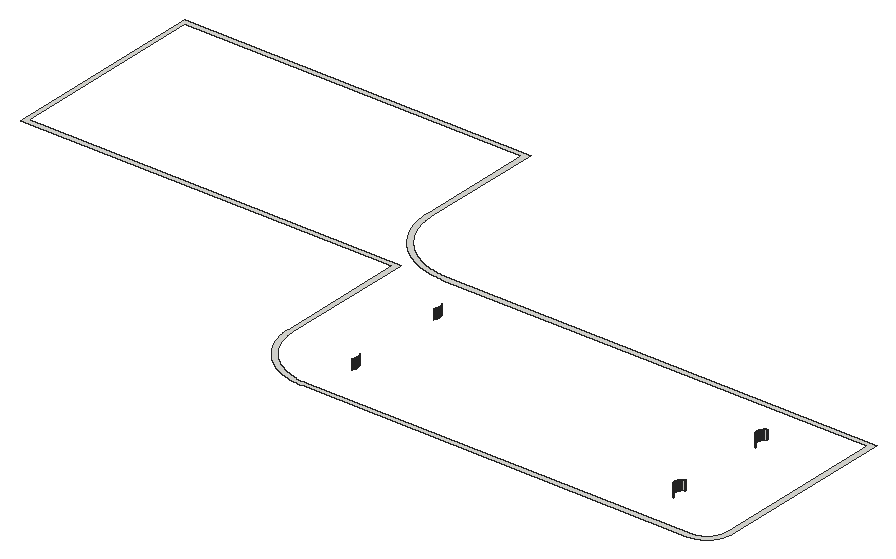
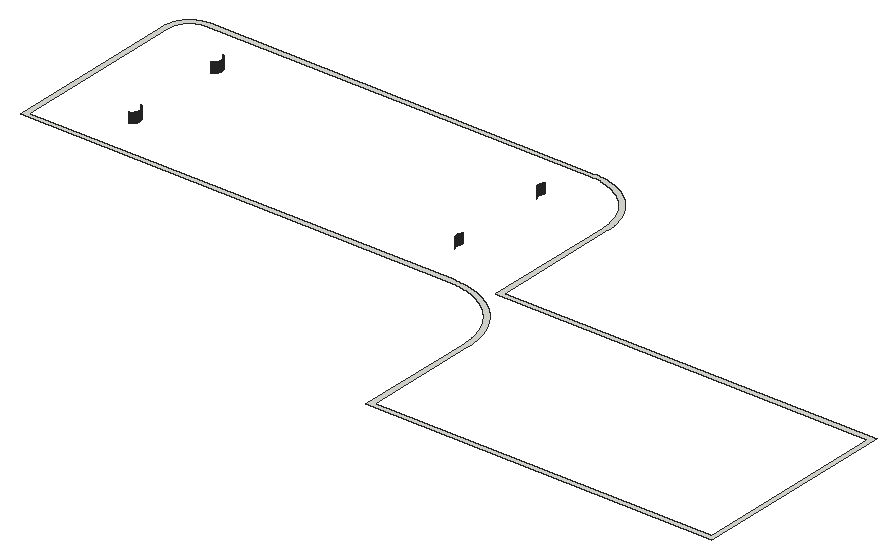
# SketchUp Ruby script. Lengths in inches.
U = 1.inch
M = Sketchup.active_model
def pt(a) = Geom::Point3d.new(a.map { |v| v * U })
def face(e, loops, mat)
  f = e.add_face(loops[0].map { |a| pt(a) })
  loops[1..].each { |l| e.add_face(l.map { |a| pt(a) }).erase! }
  f.material = f.back_material = mat if mat
  f
end
# faces: each face lists its corners as indices into pts; further lists are holes
def faces(e, pts, list, mat = nil) = list.each { |f| face(e, (f[0].is_a?(Array) ? f : [f]).map { |l| l.map { |i| pts[i] } }, mat) }
# xy, xz, yz: faces in a plane at the given z, y or x. An outline is a flat list of corners, or four numbers for a rectangle; further outlines are holes
def ring(l) = l.size == 4 ? [[l[0], l[1]], [l[2], l[1]], [l[2], l[3]], [l[0], l[3]]] : l.each_slice(2).to_a
def flat(e, list, mat, &to3) = list.each { |f| face(e, (f[0].is_a?(Array) ? f : [f]).map { |l| ring(l).map { |u, v| to3.(u, v) } }, mat) }
def xy(e, z, list, mat = nil) = flat(e, list, mat) { |x, y| [x, y, z] }
def xz(e, y, list, mat = nil) = flat(e, list, mat) { |x, z| [x, y, z] }
def yz(e, x, list, mat = nil) = flat(e, list, mat) { |y, z| [x, y, z] }
def lines(e, pts, list) = list.each { |a, b| e.add_line(pt(pts[a]), pt(pts[b])) }
# prism: a flat outline (further loops are holes) pulled along v
def prism(e, loops, v, mat = nil)
  f = face(e, loops, mat); d = Geom::Vector3d.new(v.map { |x| x * U })
  f.pushpull(f.normal.samedirection?(d) ? d.length : -d.length)
end
def box(e, o, s, mat = nil) = prism(e, [[o, [o[0] + s[0], o[1], o[2]], [o[0] + s[0], o[1] + s[1], o[2]], [o[0], o[1] + s[1], o[2]]]], [0, 0, s[2]], mat)
def at(x, y, z, deg = 0) = Geom::Transformation.translation(pt([x, y, z])) * Geom::Transformation.rotation(ORIGIN, Z_AXIS, deg.degrees)
def axes(o, x, y, z) = Geom::Transformation.new([*x, 0, *y, 0, *z, 0, *pt(o).to_a, 1])
def part(name) = M.definitions.add(name)
# library, detail: a bought-in or finely detailed component or shape, given as its bounding box
def library(name, o, s) = part(name).tap { |d| box(d.entities, o, s) }
def detail(e, o, s) = box(e.add_group.entities, o, s)
def put(e, d, t, mat = nil) = e.add_instance(d, t).tap { |i| i.material = mat if mat }
def group(e, t, mat = nil) = e.add_group.tap { |g| g.transformation = t; g.material = mat if mat }.entities
root = M.entities
xy(root,116.5,[[[157.74,124,157.48,124.01,157.21,124.02,156.69,124.04,156.43,124.0625,156.17,124.08,155.39,124.17,154.61,124.29,154.36,124.33,154.1,124.38,153.84,124.4375,153.59,124.49,153.33,124.55,153.08,124.62,152.82,124.68,152.32,124.82,151.82,124.98,151.57,125.0625,151.32,125.15,151.08,125.24,150.83,125.33,150.59,125.42,150.35,125.52,149.87,125.73,149.625,125.84,149.39,125.95,149.15,126.0625,148.92,126.18,148.6875,126.3,148.46,126.42,148,126.68,147.77,126.8125,147.55,126.95,146.89,127.37,146.67,127.52,146.46,127.67,146.24,127.82,146.03,127.97,145.82,128.13,145.62,128.29,145.41,128.46,145.01,128.79,144.8125,128.96,144.62,129.14,144.42,129.3125,144.23,129.49,144.04,129.67,143.86,129.86,143.67,130.04,143.49,130.23,143.3125,130.42,143.14,130.62,142.96,130.8125,142.79,131.01,142.46,131.41,142.29,131.62,142.13,131.82,141.97,132.03,141.82,132.24,141.67,132.46,141.52,132.67,141.37,132.89,140.95,133.55,140.8125,133.77,140.68,134,140.42,134.46,140.3,134.6875,140.18,134.92,140.0625,135.15,139.95,135.39,139.84,135.625,139.73,135.87,139.52,136.35,139.42,136.59,139.33,136.83,139.24,137.08,139.15,137.32,139.0625,137.57,138.98,137.82,138.82,138.32,138.68,138.82,138.62,139.08,138.55,139.33,138.49,139.59,138.4375,139.84,138.38,140.1,138.33,140.36,138.29,140.61,138.17,141.39,138.08,142.17,138.0625,142.43,138.04,142.69,138.02,143.21,138.01,143.48,138,143.74,138,184,22,184,22,248,130,248,130,209.73,130.01,209.47,130.01,209.2,130.03,208.9375,130.04,208.67,130.06,208.41,130.08,208.14,130.1,207.875,130.13,207.61,130.16,207.35,130.19,207.08,130.27,206.56,130.3125,206.3,130.36,206.03,130.46,205.51,130.58,204.99,130.64,204.74,130.7,204.48,130.84,203.96,130.92,203.71,131,203.45,131.16,202.95,131.43,202.2,131.53,201.95,131.625,201.7,131.73,201.46,131.83,201.21,131.9375,200.97,132.05,200.73,132.16,200.49,132.4,200.01,132.52,199.78,132.64,199.54,132.9,199.08,133.04,198.85,133.17,198.62,133.3125,198.39,133.45,198.17,133.6,197.94,133.74,197.72,133.89,197.5,134.05,197.28,134.2,197.07,134.36,196.85,134.68,196.43,134.85,196.22,135.01,196.02,135.18,195.8125,135.36,195.61,135.53,195.41,135.71,195.21,135.89,195.02,136.07,194.82,136.26,194.63,136.44,194.44,136.63,194.26,136.82,194.07,137.02,193.89,137.21,193.71,137.41,193.53,137.61,193.36,137.8125,193.18,138.02,193.01,138.22,192.85,138.43,192.68,138.85,192.36,139.07,192.2,139.28,192.05,139.5,191.89,139.72,191.74,139.94,191.6,140.17,191.45,140.39,191.3125,140.62,191.17,140.85,191.04,141.08,190.9,141.54,190.64,141.78,190.52,142.01,190.4,142.49,190.16,142.73,190.05,142.97,189.9375,143.21,189.83,143.46,189.73,143.7,189.625,143.95,189.53,144.2,189.43,144.95,189.16,145.45,189,145.71,188.92,145.96,188.84,146.48,188.7,146.74,188.64,146.99,188.58,147.51,188.46,148.03,188.36,148.3,188.3125,148.56,188.27,149.08,188.19,149.35,188.16,149.61,188.13,149.875,188.1,150.14,188.08,150.41,188.06,150.67,188.04,150.9375,188.03,151.2,188.01,151.47,188.01,151.73,188,286,188,286,131.84,285.99,131.6875,285.99,131.53,285.98,131.37,285.96,131.22,285.92,130.9,285.9,130.75,285.875,130.59,285.85,130.4375,285.8125,130.29,285.78,130.13,285.66,129.68,285.51,129.23,285.45,129.08,285.39,128.9375,285.33,128.79,285.27,128.65,285.06,128.23,284.9,127.95,284.82,127.82,284.74,127.6875,284.65,127.56,284.5625,127.43,284.47,127.3,284.38,127.17,284.28,127.05,284.18,126.92,284.08,126.8,283.98,126.6875,283.875,126.57,283.77,126.46,283.66,126.34,283.54,126.23,283.43,126.125,283.3125,126.02,283.2,125.92,283.08,125.82,282.95,125.72,282.83,125.62,282.7,125.53,282.57,125.4375,282.44,125.35,282.3125,125.26,282.18,125.18,282.05,125.1,281.77,124.94,281.35,124.73,281.21,124.67,281.0625,124.61,280.92,124.55,280.77,124.49,280.32,124.34,279.87,124.22,279.71,124.1875,279.5625,124.15,279.41,124.125,279.25,124.1,279.1,124.08,278.78,124.04,278.63,124.02,278.47,124.01,278.3125,124.01,278.16,124],[157.76,125.5,278.13,125.5,278.26,125.51,278.38,125.51,278.64,125.53,278.76,125.55,278.89,125.5625,279.02,125.58,279.14,125.6,279.27,125.625,279.39,125.65,279.52,125.68,279.76,125.74,279.89,125.78,280.25,125.9,280.37,125.95,280.49,125.99,280.6,126.04,280.72,126.1,280.84,126.15,280.95,126.21,281.0625,126.27,281.18,126.33,281.29,126.39,281.4,126.46,281.5,126.53,281.72,126.67,281.82,126.74,282.02,126.9,282.125,126.98,282.22,127.06,282.32,127.14,282.41,127.23,282.5,127.3125,282.6,127.4,282.69,127.49,282.77,127.59,282.86,127.68,282.94,127.78,283.02,127.875,283.1,127.98,283.26,128.18,283.33,128.28,283.47,128.5,283.54,128.6,283.61,128.71,283.67,128.82,283.73,128.9375,283.79,129.05,283.85,129.16,283.9,129.28,283.96,129.4,284.01,129.51,284.05,129.63,284.1,129.75,284.22,130.11,284.26,130.24,284.32,130.48,284.35,130.61,284.375,130.73,284.4,130.86,284.42,130.98,284.4375,131.11,284.45,131.24,284.47,131.36,284.49,131.62,284.49,131.74,284.5,131.87,284.5,186.5,151.71,186.5,151.15,186.52,150.86,186.53,150.58,186.54,150.3,186.5625,150.01,186.58,149.17,186.67,148.89,186.71,148.6,186.75,148.32,186.79,148.04,186.84,147.76,186.88,147.49,186.9375,147.21,186.99,146.93,187.05,146.65,187.12,146.375,187.18,146.1,187.25,145.83,187.33,145.55,187.4,145.28,187.48,145.01,187.5625,144.74,187.65,144.2,187.83,143.93,187.93,143.67,188.03,143.4,188.13,143.14,188.23,142.875,188.34,142.61,188.46,142.36,188.57,142.1,188.6875,141.84,188.81,141.58,188.93,141.33,189.0625,141.08,189.19,140.83,189.33,140.58,189.46,140.33,189.6,140.09,189.74,139.84,189.89,139.6,190.04,139.36,190.1875,139.12,190.34,138.89,190.5,138.65,190.66,138.42,190.82,138.1875,190.99,137.96,191.16,137.73,191.33,137.51,191.5,137.28,191.68,137.0625,191.86,136.85,192.04,136.63,192.22,136,192.79,135.79,192.99,135.58,193.18,135.18,193.58,134.99,193.79,134.79,194,134.22,194.63,134.04,194.85,133.86,195.0625,133.68,195.28,133.5,195.51,133.33,195.73,133.16,195.96,132.99,196.1875,132.82,196.42,132.66,196.65,132.5,196.89,132.34,197.12,132.1875,197.36,132.04,197.6,131.89,197.84,131.74,198.09,131.6,198.33,131.46,198.58,131.33,198.83,131.19,199.08,131.0625,199.33,130.93,199.58,130.81,199.84,130.6875,200.1,130.57,200.36,130.46,200.61,130.34,200.875,130.23,201.14,130.13,201.4,130.03,201.67,129.93,201.93,129.83,202.2,129.65,202.74,129.5625,203.01,129.48,203.28,129.4,203.55,129.33,203.83,129.25,204.1,129.18,204.375,129.12,204.65,129.05,204.93,128.99,205.21,128.9375,205.49,128.88,205.76,128.84,206.04,128.79,206.32,128.75,206.6,128.71,206.89,128.67,207.17,128.58,208.01,128.5625,208.3,128.54,208.58,128.53,208.86,128.52,209.15,128.51,209.43,128.5,209.72,128.5,246.5,23.5,246.5,23.5,185.5,139.5,185.5,139.5,143.76,139.51,143.52,139.51,143.27,139.53,143.03,139.54,142.79,139.6,142.07,139.69,141.35,139.81,140.63,139.86,140.39,139.9,140.15,139.96,139.92,140.01,139.68,140.07,139.45,140.13,139.21,140.19,138.98,140.26,138.75,140.33,138.51,140.41,138.28,140.48,138.05,140.5625,137.82,140.64,137.6,140.82,137.14,141,136.7,141.1,136.48,141.2,136.25,141.3,136.04,141.52,135.6,141.63,135.39,141.74,135.17,142.1,134.54,142.23,134.33,142.35,134.13,142.48,133.92,142.62,133.72,142.75,133.52,142.89,133.32,143.03,133.125,143.18,132.93,143.32,132.74,143.62,132.36,143.78,132.17,143.93,131.99,144.09,131.8,144.25,131.62,144.42,131.44,144.58,131.27,144.75,131.09,145.09,130.75,145.27,130.58,145.44,130.42,145.62,130.25,145.8,130.09,145.99,129.93,146.17,129.78,146.36,129.62,146.74,129.32,146.93,129.18,147.125,129.03,147.32,128.89,147.52,128.75,147.72,128.62,147.92,128.48,148.13,128.35,148.33,128.23,148.54,128.1,149.17,127.74,149.39,127.63,149.6,127.52,150.04,127.3,150.25,127.2,150.48,127.1,150.7,127,151.14,126.82,151.6,126.64,151.82,126.5625,152.05,126.48,152.28,126.41,152.51,126.33,152.75,126.26,152.98,126.19,153.21,126.13,153.45,126.07,153.68,126.01,153.92,125.96,154.15,125.9,154.39,125.86,154.63,125.81,155.35,125.69,156.07,125.6,156.79,125.54,157.03,125.53,157.27,125.51,157.52,125.51]]])
yz(root,162.5,[[139.84,116,139.92,119],[139.92,116,140,119],[140,116,140.08,119],[140.08,116,140.16,119],[171.84,116,171.92,119],
  [171.92,116,172,119],[172,116,172.08,119],[172.08,116,172.16,119]])
yz(root,261.5,[[139.84,116,139.92,119],[139.92,116,140,119],[140,116,140.08,119],[140.08,116,140.16,119],[171.84,116,171.92,119],
  [171.92,116,172,119],[172,116,172.08,119],[172.08,116,172.16,119]])
p = [[263.15,137.65,116],[263.08,137.68,116],[263.08,137.68,119],[263.15,137.65,119],[262.94,137.74,116],[262.86,137.77,116],
  [262.86,137.77,119],[262.94,137.74,119],[263.01,137.71,116],[263.01,137.71,119],[262.73,137.85,116],[262.66,137.89,116],
  [262.66,137.89,119],[262.73,137.85,119],[262.8,137.81,116],[262.8,137.81,119],[262.59,137.93,116],[262.53,137.98,116],
  [262.53,137.98,119],[262.59,137.93,119],[262.47,138.02,116],[262.41,138.07,116],[262.41,138.07,119],[262.47,138.02,119],
  [262.35,138.125,116],[262.29,138.18,116],[262.29,138.18,119],[262.35,138.125,119],[262.23,138.23,116],[262.18,138.29,116],
  [262.18,138.29,119],[262.23,138.23,119],[161.93,138.41,116],[161.875,138.35,116],[161.875,138.35,119],[161.93,138.41,119],
  [262.125,138.35,116],[262.07,138.41,116],[262.07,138.41,119],[262.125,138.35,119],[161.98,138.47,116],[161.98,138.47,119],
  [262.02,138.47,116],[262.02,138.47,119],[162.02,138.53,116],[162.02,138.53,119],[162.07,138.59,116],[162.07,138.59,119],
  [261.98,138.53,116],[261.93,138.59,116],[261.93,138.59,119],[261.98,138.53,119],[162.11,138.66,116],[162.11,138.66,119],
  [261.89,138.66,116],[261.89,138.66,119],[162.15,138.73,116],[162.15,138.73,119],[162.19,138.8,116],[162.19,138.8,119],
  [261.85,138.73,116],[261.81,138.8,116],[261.81,138.8,119],[261.85,138.73,119],[162.23,138.87,116],[162.23,138.87,119],
  [261.77,138.87,116],[261.77,138.87,119],[162.26,138.9375,116],[162.26,138.9375,119],[162.29,139.01,116],[162.29,139.01,119],
  [261.74,138.9375,116],[261.71,139.01,116],[261.71,139.01,119],[261.74,138.9375,119],[162.32,139.08,116],[162.32,139.08,119],
  [261.68,139.08,116],[261.68,139.08,119],[162.35,139.15,116],[162.35,139.15,119],[261.65,139.15,116],[261.65,139.15,119],
  [162.38,139.23,116],[162.38,139.23,119],[162.4,139.3,116],[162.4,139.3,119],[261.62,139.23,116],[261.6,139.3,116],
  [261.6,139.3,119],[261.62,139.23,119],[162.42,139.38,116],[162.42,139.38,119],[261.58,139.38,116],[261.58,139.38,119],
  [162.44,139.45,116],[162.44,139.45,119],[261.56,139.45,116],[261.56,139.45,119],[162.46,139.53,116],[162.46,139.53,119],
  [162.47,139.61,116],[162.47,139.61,119],[261.54,139.53,116],[261.53,139.61,116],[261.53,139.61,119],[261.54,139.53,119],
  [162.48,139.6875,116],[162.48,139.6875,119],[261.52,139.6875,116],[261.52,139.6875,119],[162.49,139.76,116],[162.49,139.76,119],
  [261.51,139.76,116],[261.51,139.76,119],[162.5,139.84,116],[162.5,139.84,119],[261.5,139.84,116],[261.5,139.84,119],
  [162.48,140.3125,116],[162.49,140.24,116],[162.49,140.24,119],[162.48,140.3125,119],[162.5,140.16,116],[162.5,140.16,119],
  [261.5,140.16,116],[261.51,140.24,116],[261.51,140.24,119],[261.5,140.16,119],[261.52,140.3125,116],[261.52,140.3125,119],
  [162.47,140.39,116],[162.47,140.39,119],[261.53,140.39,116],[261.53,140.39,119],[162.46,140.47,116],[162.46,140.47,119],
  [261.54,140.47,116],[261.54,140.47,119],[162.42,140.62,116],[162.44,140.55,116],[162.44,140.55,119],[162.42,140.62,119],
  [261.56,140.55,116],[261.56,140.55,119],[261.58,140.62,116],[261.58,140.62,119],[162.4,140.7,116],[162.4,140.7,119],
  [261.6,140.7,116],[261.6,140.7,119],[162.38,140.77,116],[162.38,140.77,119],[261.62,140.77,116],[261.62,140.77,119],
  [162.32,140.92,116],[162.35,140.85,116],[162.35,140.85,119],[162.32,140.92,119],[261.65,140.85,116],[261.65,140.85,119],
  [261.68,140.92,116],[261.68,140.92,119],[162.29,140.99,116],[162.29,140.99,119],[261.71,140.99,116],[261.71,140.99,119],
  [162.26,141.0625,116],[162.26,141.0625,119],[261.74,141.0625,116],[261.74,141.0625,119],[162.19,141.2,116],[162.23,141.13,116],
  [162.23,141.13,119],[162.19,141.2,119],[261.77,141.13,116],[261.77,141.13,119],[261.81,141.2,116],[261.81,141.2,119],
  [162.15,141.27,116],[162.15,141.27,119],[261.85,141.27,116],[261.85,141.27,119],[162.07,141.41,116],[162.11,141.34,116],
  [162.11,141.34,119],[162.07,141.41,119],[261.89,141.34,116],[261.89,141.34,119],[261.93,141.41,116],[261.93,141.41,119],
  [162.02,141.47,116],[162.02,141.47,119],[261.98,141.47,116],[261.98,141.47,119],[161.93,141.59,116],[161.98,141.53,116],
  [161.98,141.53,119],[161.93,141.59,119],[262.02,141.53,116],[262.02,141.53,119],[262.07,141.59,116],[262.07,141.59,119],
  [161.875,141.65,116],[161.875,141.65,119],[262.125,141.65,116],[262.125,141.65,119],[161.82,141.71,116],[161.82,141.71,119],
  [262.18,141.71,116],[262.18,141.71,119],[262.23,141.77,116],[262.23,141.77,119],[262.29,141.82,116],[262.29,141.82,119],
  [262.35,141.875,116],[262.35,141.875,119],[262.41,141.93,116],[262.41,141.93,119],[262.47,141.98,116],[262.47,141.98,119],
  [262.53,142.02,116],[262.53,142.02,119],[262.59,142.07,116],[262.59,142.07,119],[262.66,142.11,116],[262.66,142.11,119],
  [262.73,142.15,116],[262.73,142.15,119],[262.8,142.19,116],[262.8,142.19,119],[262.86,142.23,116],[262.86,142.23,119],
  [262.94,142.26,116],[262.94,142.26,119],[263.01,142.29,116],[263.01,142.29,119],[263.08,142.32,116],[263.08,142.32,119],
  [262.94,169.74,116],[262.86,169.77,116],[262.86,169.77,119],[262.94,169.74,119],[263.01,169.71,116],[263.01,169.71,119],
  [263.08,169.68,116],[263.08,169.68,119],[262.73,169.85,116],[262.66,169.89,116],[262.66,169.89,119],[262.73,169.85,119],
  [262.8,169.81,116],[262.8,169.81,119],[262.59,169.93,116],[262.53,169.98,116],[262.53,169.98,119],[262.59,169.93,119],
  [262.47,170.02,116],[262.41,170.07,116],[262.41,170.07,119],[262.47,170.02,119],[262.35,170.125,116],[262.29,170.18,116],
  [262.29,170.18,119],[262.35,170.125,119],[262.23,170.23,116],[262.18,170.29,116],[262.18,170.29,119],[262.23,170.23,119],
  [161.93,170.41,116],[161.875,170.35,116],[161.875,170.35,119],[161.93,170.41,119],[262.125,170.35,116],[262.07,170.41,116],
  [262.07,170.41,119],[262.125,170.35,119],[161.98,170.47,116],[161.98,170.47,119],[262.02,170.47,116],[262.02,170.47,119],
  [162.02,170.53,116],[162.02,170.53,119],[162.07,170.59,116],[162.07,170.59,119],[261.98,170.53,116],[261.93,170.59,116],
  [261.93,170.59,119],[261.98,170.53,119],[162.11,170.66,116],[162.11,170.66,119],[261.89,170.66,116],[261.89,170.66,119],
  [162.15,170.73,116],[162.15,170.73,119],[162.19,170.8,116],[162.19,170.8,119],[261.85,170.73,116],[261.81,170.8,116],
  [261.81,170.8,119],[261.85,170.73,119],[162.23,170.87,116],[162.23,170.87,119],[261.77,170.87,116],[261.77,170.87,119],
  [162.26,170.9375,116],[162.26,170.9375,119],[162.29,171.01,116],[162.29,171.01,119],[261.74,170.9375,116],[261.71,171.01,116],
  [261.71,171.01,119],[261.74,170.9375,119],[162.32,171.08,116],[162.32,171.08,119],[261.68,171.08,116],[261.68,171.08,119],
  [162.35,171.15,116],[162.35,171.15,119],[261.65,171.15,116],[261.65,171.15,119],[162.38,171.23,116],[162.38,171.23,119],
  [162.4,171.3,116],[162.4,171.3,119],[261.62,171.23,116],[261.6,171.3,116],[261.6,171.3,119],[261.62,171.23,119],
  [162.42,171.38,116],[162.42,171.38,119],[261.58,171.38,116],[261.58,171.38,119],[162.44,171.45,116],[162.44,171.45,119],
  [261.56,171.45,116],[261.56,171.45,119],[162.46,171.53,116],[162.46,171.53,119],[162.47,171.61,116],[162.47,171.61,119],
  [261.54,171.53,116],[261.53,171.61,116],[261.53,171.61,119],[261.54,171.53,119],[162.48,171.6875,116],[162.48,171.6875,119],
  [261.52,171.6875,116],[261.52,171.6875,119],[162.49,171.76,116],[162.49,171.76,119],[261.51,171.76,116],[261.51,171.76,119],
  [162.5,171.84,116],[162.5,171.84,119],[261.5,171.84,116],[261.5,171.84,119],[162.48,172.3125,116],[162.49,172.24,116],
  [162.49,172.24,119],[162.48,172.3125,119],[162.5,172.16,116],[162.5,172.16,119],[261.5,172.16,116],[261.51,172.24,116],
  [261.51,172.24,119],[261.5,172.16,119],[261.52,172.3125,116],[261.52,172.3125,119],[162.47,172.39,116],[162.47,172.39,119],
  [261.53,172.39,116],[261.53,172.39,119],[162.46,172.47,116],[162.46,172.47,119],[261.54,172.47,116],[261.54,172.47,119],
  [162.42,172.62,116],[162.44,172.55,116],[162.44,172.55,119],[162.42,172.62,119],[261.56,172.55,116],[261.56,172.55,119],
  [261.58,172.62,116],[261.58,172.62,119],[162.4,172.7,116],[162.4,172.7,119],[261.6,172.7,116],[261.6,172.7,119],
  [162.38,172.77,116],[162.38,172.77,119],[261.62,172.77,116],[261.62,172.77,119],[162.32,172.92,116],[162.35,172.85,116],
  [162.35,172.85,119],[162.32,172.92,119],[261.65,172.85,116],[261.65,172.85,119],[261.68,172.92,116],[261.68,172.92,119],
  [162.29,172.99,116],[162.29,172.99,119],[261.71,172.99,116],[261.71,172.99,119],[162.26,173.0625,116],[162.26,173.0625,119],
  [261.74,173.0625,116],[261.74,173.0625,119],[162.19,173.2,116],[162.23,173.13,116],[162.23,173.13,119],[162.19,173.2,119],
  [261.77,173.13,116],[261.77,173.13,119],[261.81,173.2,116],[261.81,173.2,119],[162.15,173.27,116],[162.15,173.27,119],
  [261.85,173.27,116],[261.85,173.27,119],[162.07,173.41,116],[162.11,173.34,116],[162.11,173.34,119],[162.07,173.41,119],
  [261.89,173.34,116],[261.89,173.34,119],[261.93,173.41,116],[261.93,173.41,119],[162.02,173.47,116],[162.02,173.47,119],
  [261.98,173.47,116],[261.98,173.47,119],[161.93,173.59,116],[161.98,173.53,116],[161.98,173.53,119],[161.93,173.59,119],
  [262.02,173.53,116],[262.02,173.53,119],[262.07,173.59,116],[262.07,173.59,119],[161.875,173.65,116],[161.875,173.65,119],
  [262.125,173.65,116],[262.125,173.65,119],[262.18,173.71,116],[262.18,173.71,119],[262.23,173.77,116],[262.23,173.77,119],
  [262.29,173.82,116],[262.29,173.82,119],[262.35,173.875,116],[262.35,173.875,119],[262.41,173.93,116],[262.41,173.93,119],
  [262.47,173.98,116],[262.47,173.98,119],[262.53,174.02,116],[262.53,174.02,119],[262.59,174.07,116],[262.59,174.07,119],
  [262.66,174.11,116],[262.66,174.11,119],[262.73,174.15,116],[262.73,174.15,119],[262.8,174.19,116],[262.8,174.19,119],
  [262.86,174.23,116],[262.86,174.23,119],[262.94,174.26,116],[262.94,174.26,119],[263.01,174.29,116],[263.01,174.29,119],
  [263.08,174.32,116],[263.08,174.32,119]]
faces(root,p,[[0,1,2,3],[4,5,6,7],[8,4,7,9],[1,8,9,2],[10,11,12,13],[14,10,13,15],[5,14,15,6],[16,17,18,19],
  [11,16,19,12],[20,21,22,23],[17,20,23,18],[24,25,26,27],[21,24,27,22],[28,29,30,31],[25,28,31,26],[32,33,34,35],
  [36,37,38,39],[29,36,39,30],[40,32,35,41],[37,42,43,38],[44,40,41,45],[46,44,45,47],[48,49,50,51],[42,48,51,43],
  [52,46,47,53],[49,54,55,50],[56,52,53,57],[58,56,57,59],[60,61,62,63],[54,60,63,55],[64,58,59,65],[61,66,67,62],
  [68,64,65,69],[70,68,69,71],[72,73,74,75],[66,72,75,67],[76,70,71,77],[73,78,79,74],[80,76,77,81],[78,82,83,79],
  [84,80,81,85],[86,84,85,87],[88,89,90,91],[82,88,91,83],[92,86,87,93],[89,94,95,90],[96,92,93,97],[94,98,99,95],
  [100,96,97,101],[102,100,101,103],[104,105,106,107],[98,104,107,99],[108,102,103,109],[105,110,111,106],[112,108,109,113],[110,114,115,111],
  [116,112,113,117],[114,118,119,115],[120,121,122,123],[121,124,125,122],[126,127,128,129],[127,130,131,128],[132,120,123,133],[130,134,135,131],
  [136,132,133,137],[134,138,139,135],[140,141,142,143],[141,136,137,142],[138,144,145,139],[144,146,147,145],[148,140,143,149],[146,150,151,147],
  [152,148,149,153],[150,154,155,151],[156,157,158,159],[157,152,153,158],[154,160,161,155],[160,162,163,161],[164,156,159,165],[162,166,167,163],
  [168,164,165,169],[166,170,171,167],[172,173,174,175],[173,168,169,174],[170,176,177,171],[176,178,179,177],[180,172,175,181],[178,182,183,179],
  [184,185,186,187],[185,180,181,186],[182,188,189,183],[188,190,191,189],[192,184,187,193],[190,194,195,191],[196,197,198,199],[197,192,193,198],
  [194,200,201,195],[200,202,203,201],[204,196,199,205],[202,206,207,203],[208,204,205,209],[206,210,211,207],[210,212,213,211],[212,214,215,213],
  [214,216,217,215],[216,218,219,217],[218,220,221,219],[220,222,223,221],[222,224,225,223],[224,226,227,225],[226,228,229,227],[228,230,231,229],
  [230,232,233,231],[232,234,235,233],[234,236,237,235],[236,238,239,237],[240,241,242,243],[244,240,243,245],[246,244,245,247],[248,249,250,251],
  [252,248,251,253],[241,252,253,242],[254,255,256,257],[249,254,257,250],[258,259,260,261],[255,258,261,256],[262,263,264,265],[259,262,265,260],
  [266,267,268,269],[263,266,269,264],[270,271,272,273],[274,275,276,277],[267,274,277,268],[278,270,273,279],[275,280,281,276],[282,278,279,283],
  [284,282,283,285],[286,287,288,289],[280,286,289,281],[290,284,285,291],[287,292,293,288],[294,290,291,295],[296,294,295,297],[298,299,300,301],
  [292,298,301,293],[302,296,297,303],[299,304,305,300],[306,302,303,307],[308,306,307,309],[310,311,312,313],[304,310,313,305],[314,308,309,315],
  [311,316,317,312],[318,314,315,319],[316,320,321,317],[322,318,319,323],[324,322,323,325],[326,327,328,329],[320,326,329,321],[330,324,325,331],
  [327,332,333,328],[334,330,331,335],[332,336,337,333],[338,334,335,339],[340,338,339,341],[342,343,344,345],[336,342,345,337],[346,340,341,347],
  [343,348,349,344],[350,346,347,351],[348,352,353,349],[354,350,351,355],[352,356,357,353],[358,359,360,361],[359,362,363,360],[364,365,366,367],
  [365,368,369,366],[370,358,361,371],[368,372,373,369],[374,370,371,375],[372,376,377,373],[378,379,380,381],[379,374,375,380],[376,382,383,377],
  [382,384,385,383],[386,378,381,387],[384,388,389,385],[390,386,387,391],[388,392,393,389],[394,395,396,397],[395,390,391,396],[392,398,399,393],
  [398,400,401,399],[402,394,397,403],[400,404,405,401],[406,402,403,407],[404,408,409,405],[410,411,412,413],[411,406,407,412],[408,414,415,409],
  [414,416,417,415],[418,410,413,419],[416,420,421,417],[422,423,424,425],[423,418,419,424],[420,426,427,421],[426,428,429,427],[430,422,425,431],
  [428,432,433,429],[434,435,436,437],[435,430,431,436],[432,438,439,433],[438,440,441,439],[442,434,437,443],[440,444,445,441],[444,446,447,445],
  [446,448,449,447],[448,450,451,449],[450,452,453,451],[452,454,455,453],[454,456,457,455],[456,458,459,457],[458,460,461,459],[460,462,463,461],
  [462,464,465,463],[464,466,467,465],[466,468,469,467],[468,470,471,469],[470,472,473,471],[472,474,475,473]])
